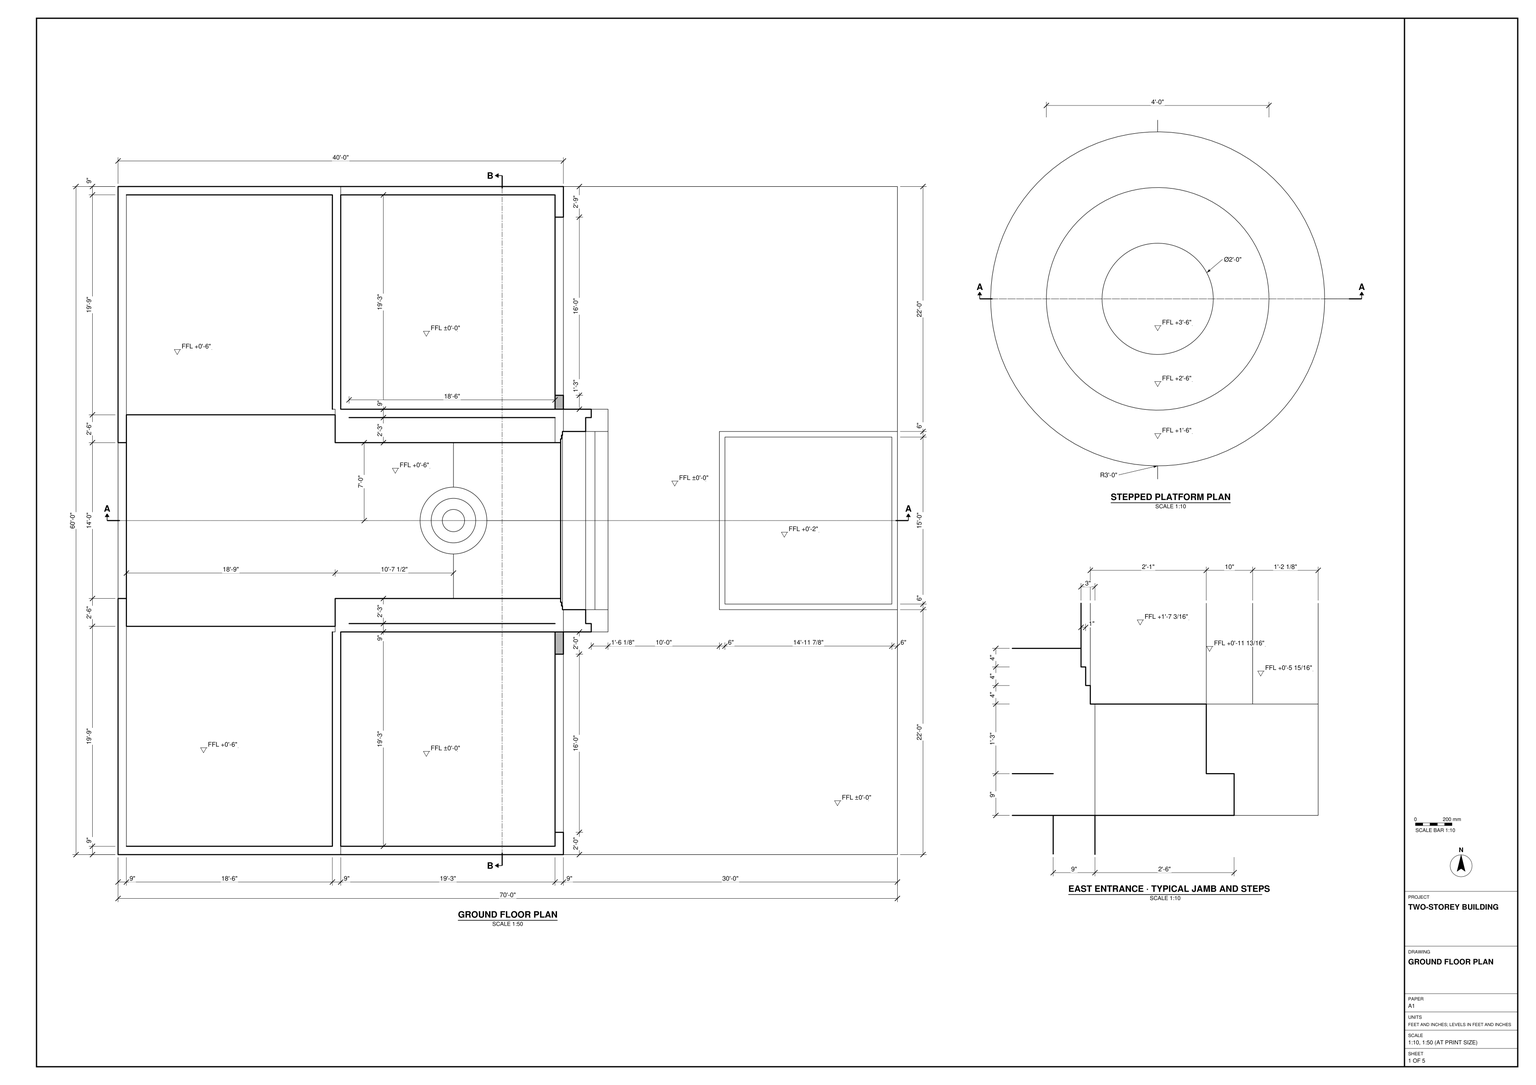
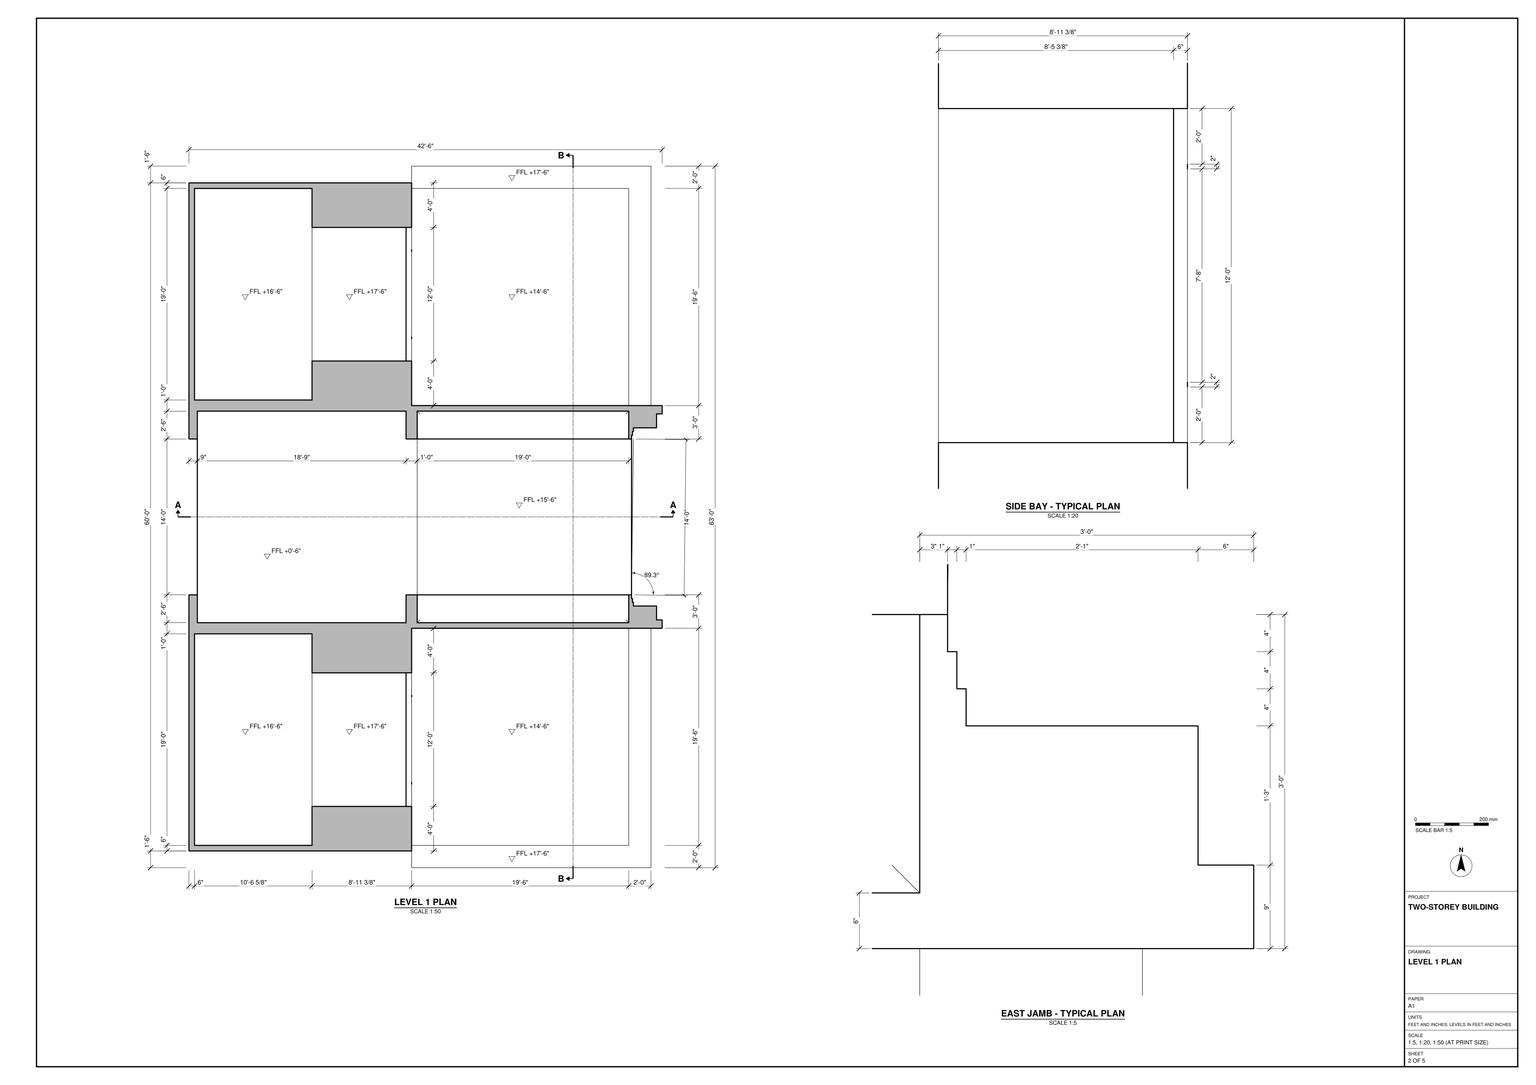
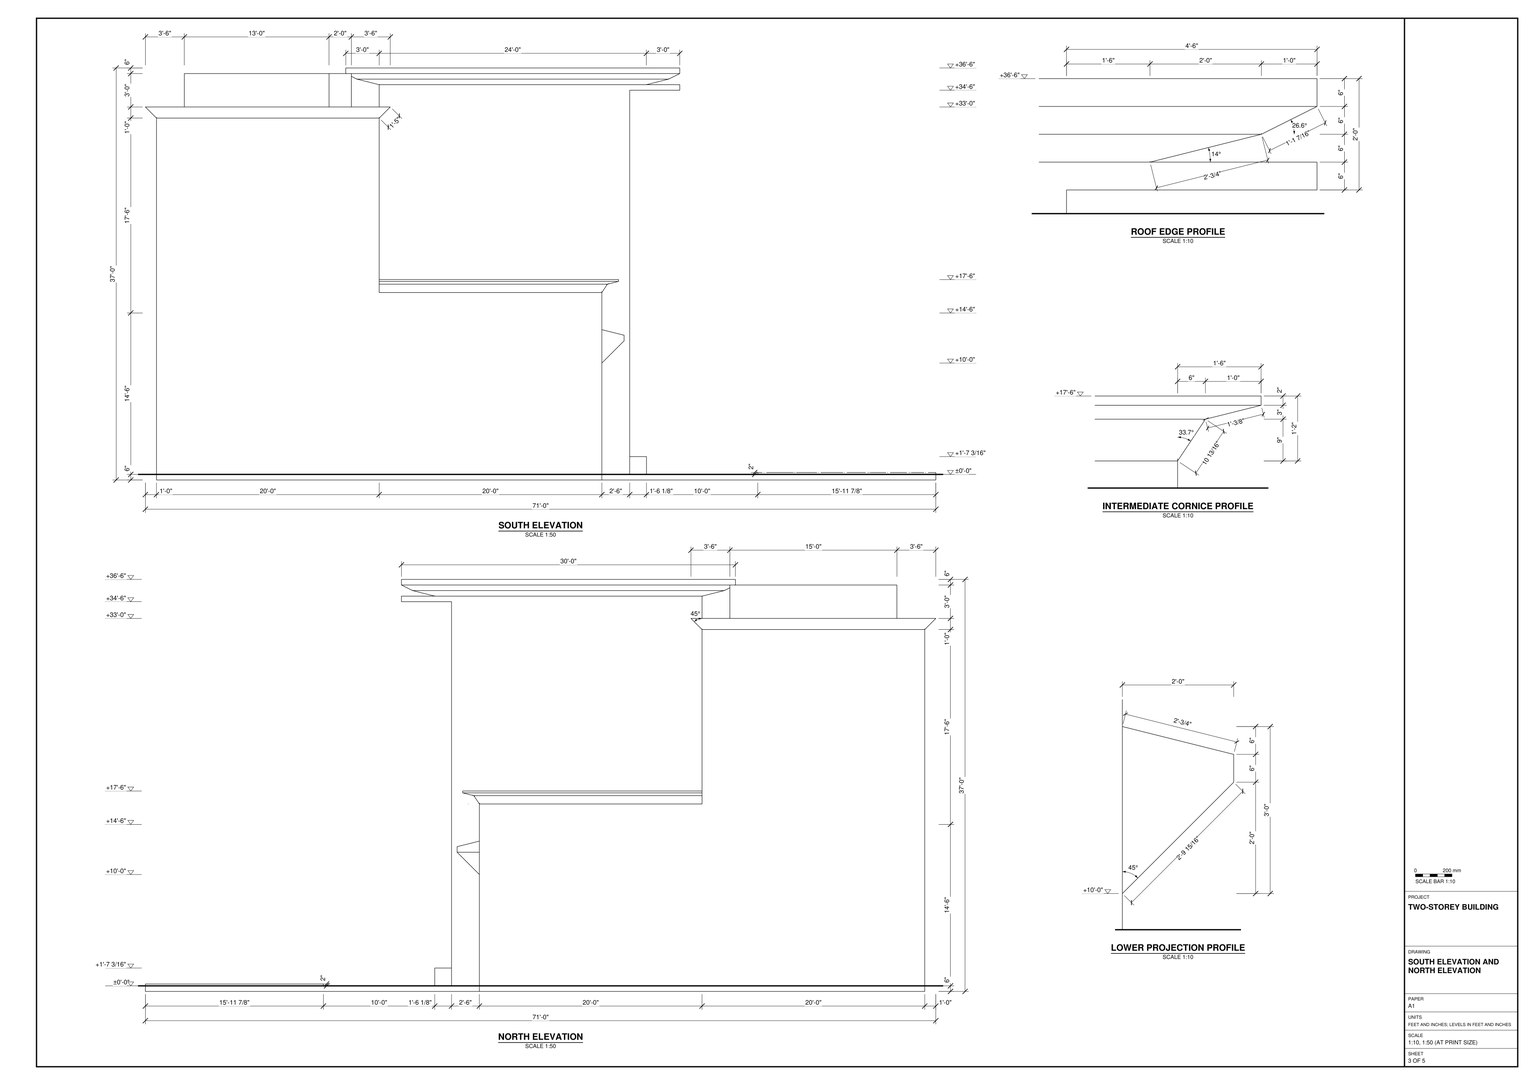
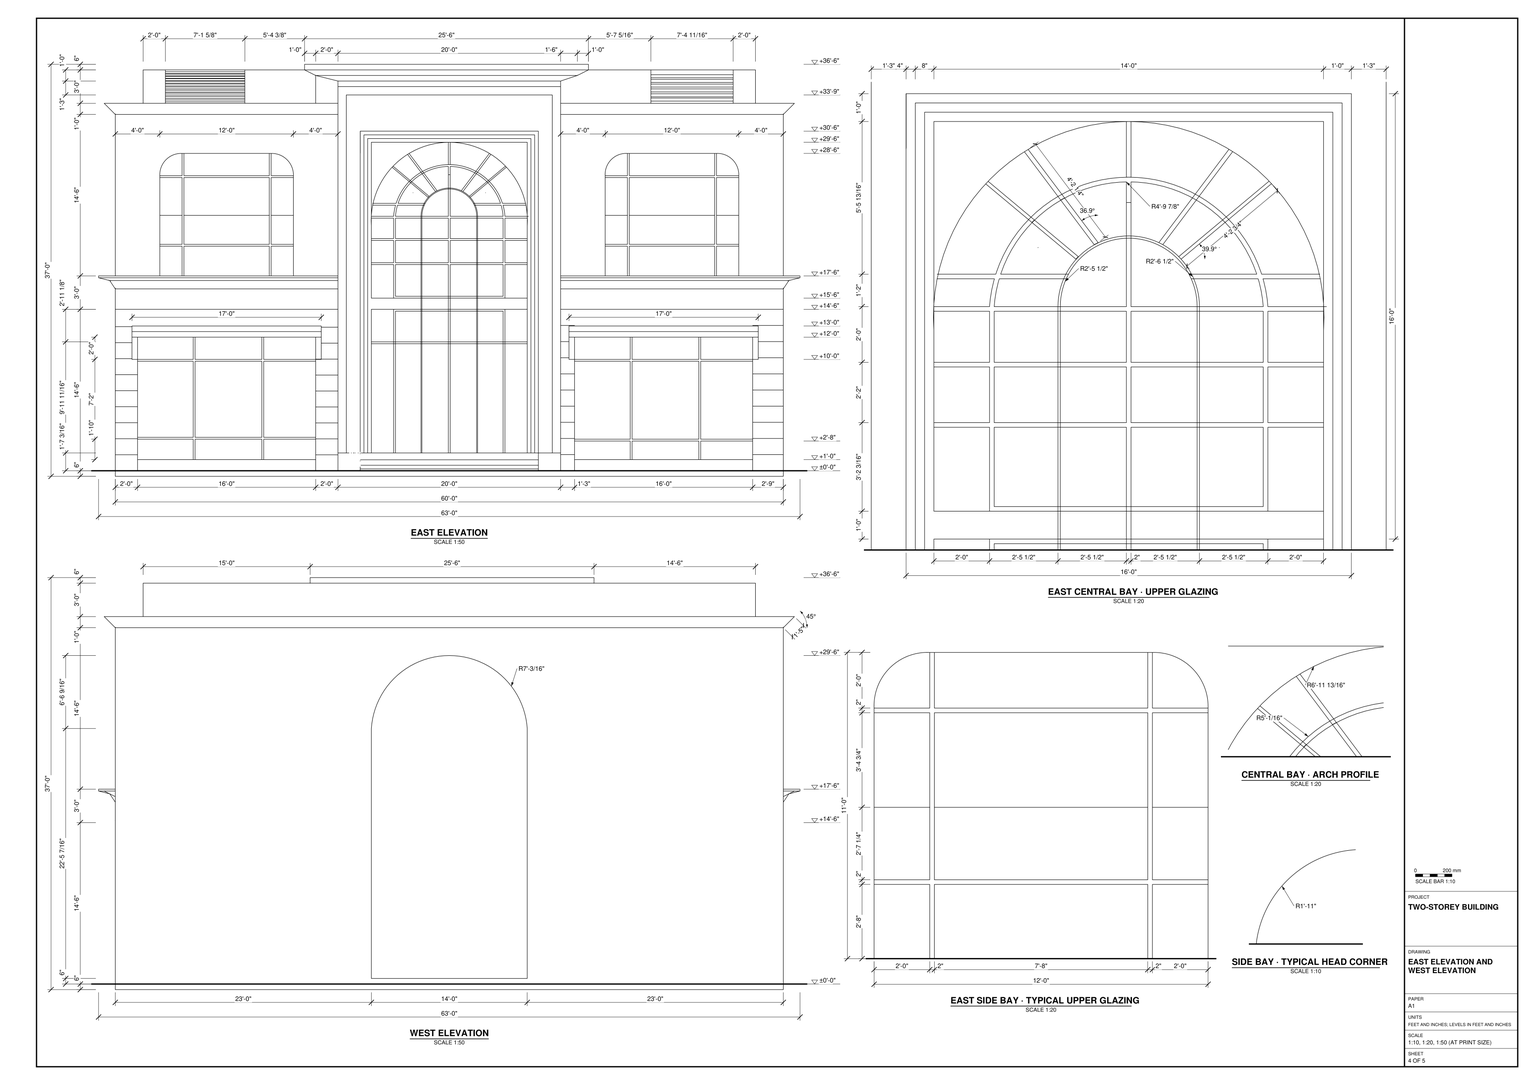
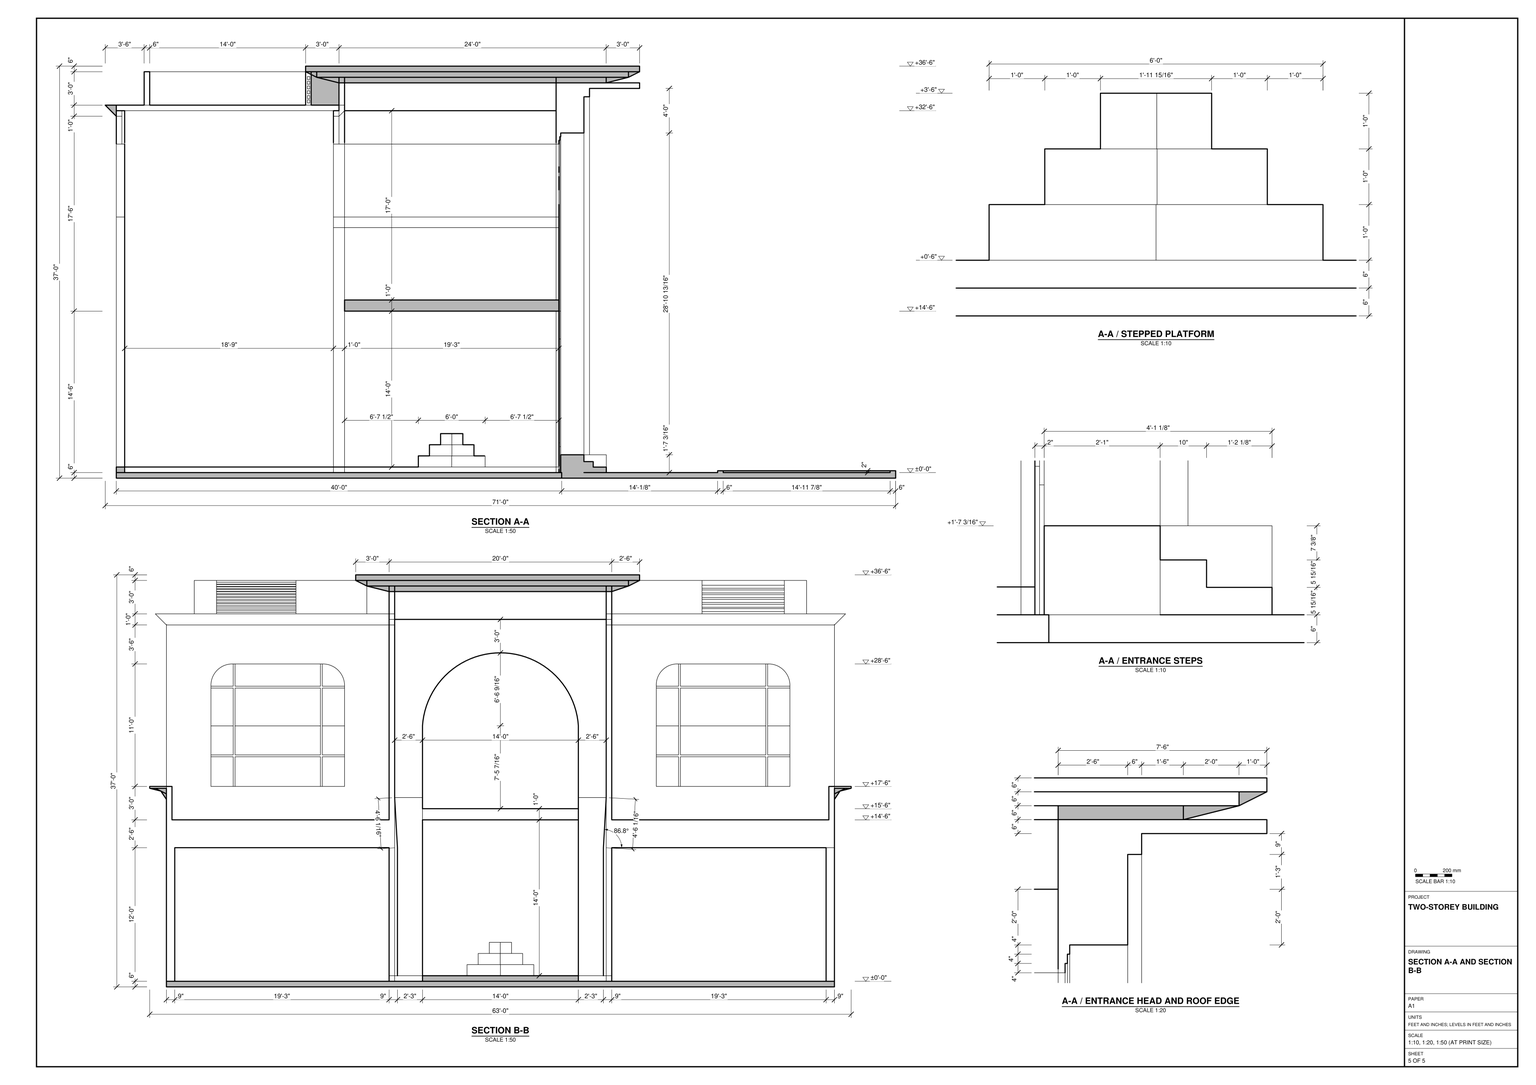
Build the two-storey building and its east forecourt in SketchUp using task_files/diagram_01.pdf. Work in feet and inches. The complete model shall measure 71'-0" east to west, 63'-0" north to south and 37'-0" from base to highest roof edge. Set the ground-floor datum at ±0'-0" and the upper-storey reference level at +14'-6". Follow the local floor levels marked on the plans rather than setting every slab on a storey at the same height.

Lay out the central east–west space with a pair of rooms on either side. Build the walls at their drawn thicknesses and retain the openings shown in plan. Align the concentric tiers of the circular platform with the east entrance. Model the entrance steps, profiled jambs and rectangular raised area across the forecourt. On the upper storey, distinguish the slab over the eastern part of the central space from the opening to the floor below. Follow the side-bay detail on both sides. Use the elevations and enlarged profiles to shape the roof edges, intermediate cornices and lower projections.

Keep walls, slabs, roof elements and each furniture or joinery piece shown in separate groups or components, and use components for repeated parts. Any decor or loose items shown may use suitable library components. Save one SketchUp model as output_files/two_storey_building_with_a_circular_stepped_platform.skp.

# SketchUp Ruby script. Lengths in inches.
U = 1.inch
M = Sketchup.active_model
def pt(a) = Geom::Point3d.new(a.map { |v| v * U })
def face(e, loops, mat)
  f = e.add_face(loops[0].map { |a| pt(a) })
  loops[1..].each { |l| e.add_face(l.map { |a| pt(a) }).erase! }
  f.material = f.back_material = mat if mat
  f
end
# faces: each face lists its corners as indices into pts; further lists are holes
def faces(e, pts, list, mat = nil) = list.each { |f| face(e, (f[0].is_a?(Array) ? f : [f]).map { |l| l.map { |i| pts[i] } }, mat) }
# xy, xz, yz: faces in a plane at the given z, y or x. An outline is a flat list of corners, or four numbers for a rectangle; further outlines are holes
def ring(l) = l.size == 4 ? [[l[0], l[1]], [l[2], l[1]], [l[2], l[3]], [l[0], l[3]]] : l.each_slice(2).to_a
def flat(e, list, mat, &to3) = list.each { |f| face(e, (f[0].is_a?(Array) ? f : [f]).map { |l| ring(l).map { |u, v| to3.(u, v) } }, mat) }
def xy(e, z, list, mat = nil) = flat(e, list, mat) { |x, y| [x, y, z] }
def xz(e, y, list, mat = nil) = flat(e, list, mat) { |x, z| [x, y, z] }
def yz(e, x, list, mat = nil) = flat(e, list, mat) { |y, z| [x, y, z] }
def lines(e, pts, list) = list.each { |a, b| e.add_line(pt(pts[a]), pt(pts[b])) }
# prism: a flat outline (further loops are holes) pulled along v
def prism(e, loops, v, mat = nil)
  f = face(e, loops, mat); d = Geom::Vector3d.new(v.map { |x| x * U })
  f.pushpull(f.normal.samedirection?(d) ? d.length : -d.length)
end
def box(e, o, s, mat = nil) = prism(e, [[o, [o[0] + s[0], o[1], o[2]], [o[0] + s[0], o[1] + s[1], o[2]], [o[0], o[1] + s[1], o[2]]]], [0, 0, s[2]], mat)
def at(x, y, z, deg = 0) = Geom::Transformation.translation(pt([x, y, z])) * Geom::Transformation.rotation(ORIGIN, Z_AXIS, deg.degrees)
def axes(o, x, y, z) = Geom::Transformation.new([*x, 0, *y, 0, *z, 0, *pt(o).to_a, 1])
def part(name) = M.definitions.add(name)
# library, detail: a bought-in or finely detailed component or shape, given as its bounding box
def library(name, o, s) = part(name).tap { |d| box(d.entities, o, s) }
def detail(e, o, s) = box(e.add_group.entities, o, s)
def put(e, d, t, mat = nil) = e.add_instance(d, t).tap { |i| i.material = mat if mat }
def group(e, t, mat = nil) = e.add_group.tap { |g| g.transformation = t; g.material = mat if mat }.entities
root = M.entities
M.materials.add("D01_Frost_White").color = [255, 242, 206]
M.materials.add("LightPink_Translucent").color = [144, 107, 117]
M.materials.add("ThomThom - Hat2").color = [38, 38, 38]
c1 = part("blade")
p = [[2.15,0.21,22],[0,0.17,0],[0.09,0.45,0],[2.18,0.31,22],[2.29,0.31,22],[0.38,0.45,0],
  [2.48,0.24,33],[2.49,0.24,33],[2.48,0.22,33]]
faces(c1.entities,p,[[0,1,2,3],[4,5,2,3],[6,3,4,7],[8,0,3,6]])
c2 = part("seeds")
p = [[0.3,-0.1,1.38],[-0.01,-0.03,1.59],[-0.01,-0.03,0.03],[0.14,-0.07,-0.07],[0.29,-0.03,3],[0.15,0.01,3.11]]
faces(c2.entities,p,[[0,1,2,3],[1,0,4,5]],"LightPink_Translucent")
c3 = part("blade with seeds")
put(c3.entities,c1,at(0,0,0))
put(c3.entities,c2,axes([2.4,0.25,30.99],[1.5799,-0.05474,1.17369],[-0.12525,1.92788,0.29478],[-0.07173,-0.02425,1.56792]))
c4 = part("Regal mist grass")
put(c4.entities,c3,axes([-3.26,-3.84,1.05],[0.05632,0.08194,0.78597],[-0.27153,0.73654,-0.07427],[-0.27499,0.00533,0.13909]))
put(c4.entities,c3,axes([-3.73,-1.59,0.19],[0.48504,-0.05875,0.50893],[-0.30767,0.51765,0.37393],[-0.23969,-0.07765,0.1121]))
put(c4.entities,c3,axes([-2.85,-2.28,0.11],[0.14833,0.22859,0.63362],[-0.3418,0.62134,-0.13627],[-0.35096,-0.14851,0.27091]))
put(c4.entities,c3,axes([3.2,1.81,0.97],[0.43228,0.51405,-0.15691],[-0.49359,0.48662,0.20258],[0.25079,0.07404,0.38762]))
put(c4.entities,c3,axes([2.7,2.1,0.19],[-0.42777,-0.23608,0.50893],[0.55235,-0.23987,0.37393],[0.14898,0.20319,0.1121]))
put(c4.entities,c3,axes([2.71,1.87,1.19],[0.04068,-0.83498,-0.05388],[0.77022,0.02282,-0.29906],[0.29664,0.058,0.45442]))
put(c4.entities,c3,axes([-3.45,-1.04,0.97],[-0.63139,-0.22904,-0.15691],[0.18416,-0.66822,0.20258],[-0.25421,0.06127,0.38762]))
put(c4.entities,c3,axes([-0.36,0.56,0.04],[0.20136,-0.97289,-0.10381],[0.95476,0.16959,0.22717],[-0.16683,-0.13435,0.69317]))
put(c4.entities,c3,axes([-2.43,-0.5,0.06],[0,0.82104,0.22],[-0.85,0,0],[0,-0.187,0.69788]))
put(c4.entities,c3,axes([1.82,-1.29,-0.13],[0.7903,0.13461,-0.27628],[-0.16677,0.83032,-0.07251],[0.23585,0.10061,0.60984]))
put(c4.entities,c3,axes([2.42,-3.36,0.01],[0.475,-0.82272,0],[0.79469,0.45881,-0.22867],[0.181,0.1045,0.72539]))
put(c4.entities,c3,axes([-2,3.05,0.45],[0.01669,-0.42385,0.68389],[0.75077,0.22388,0.09451],[-0.06505,0.45172,0.32293]))
put(c4.entities,c3,axes([-0.36,3.06,1.2],[-0.74862,-0.21464,0.23609],[0.25599,-0.70567,0.19467],[0.04499,0.27751,0.48853]))
put(c4.entities,c3,axes([-0.35,2.54,1.2],[0.22904,-0.63139,0.15691],[0.66822,0.18416,-0.20258],[0.06127,0.25421,0.38762]))
put(c4.entities,c3,axes([0.87,-4.07,1.06],[0.74862,0.21464,0.21269],[-0.25599,0.70567,0.17538],[-0.04499,-0.27751,0.44012]))
put(c4.entities,c3,axes([0.86,-3.55,1.2],[-0.22904,0.63139,0.15691],[-0.66822,-0.18416,-0.20258],[-0.06127,-0.25421,0.38762]))
put(c4.entities,c3,axes([-2.31,3.6875,0.11],[0.23975,-0.12952,0.63362],[0.59193,0.39053,-0.13627],[-0.17618,0.33792,0.27091]))
put(c4.entities,c3,axes([-0.89,-5.97,1.05],[-0.01417,0.09841,0.78597],[-0.69904,0.35716,-0.07427],[-0.20571,-0.18257,0.13909]))
put(c4.entities,c3,axes([2.82,2.98,-0.38],[0.05535,-0.11853,0.78135],[0.69686,-0.3491,-0.11937],[0.21127,0.18068,0.13309]))
put(c4.entities,c3,axes([0.6,3.36,1.05],[0.00225,-0.0994,0.78597],[0.65107,-0.43855,-0.07427],[0.22615,0.15653,0.13909]))
put(c4.entities,c3,axes([3.04,1.81,1.06],[-0.56019,0.541,0.21269],[-0.48313,-0.57453,0.17538],[0.26282,0.09979,0.44012]))
put(c4.entities,c3,axes([2.59,1.54,1.2],[-0.43228,-0.51405,0.15691],[0.49359,-0.48662,-0.20258],[0.25079,0.07404,0.38762]))
put(c4.entities,c3,axes([2.85,-2.86,-0.15],[0.71104,0.41052,-0.22],[-0.425,0.73612,0],[0.16194,0.0935,0.69788]))
put(c4.entities,c3,axes([-3.85,-0.6,1.05],[-0.12406,0.1066,0.77516],[0.01055,0.77884,-0.12259],[-0.28438,0.10128,0.06217]))
put(c4.entities,c3,axes([1.3,0.61,0.12],[0.56129,0.4933,0.06416],[-0.46819,0.55654,-0.18321],[-0.13032,0.07524,0.56159]))
put(c4.entities,c3,axes([1.125,0.43,0.14],[0.08853,0.93685,-0.12892],[-0.92207,0.05665,-0.22156],[-0.16237,0.12479,0.70765]))
put(c4.entities,c3,axes([-0.48,-0.93,-0.06],[0.36861,-0.73982,-0.19823],[0.76592,0.35605,0.0954],[0,-0.17054,0.63647]))
put(c4.entities,c3,axes([-3.05,-1.34,1.19],[0.38226,0.74345,-0.05388],[-0.67844,0.36535,-0.29906],[-0.2859,0.09809,0.45442]))
put(c4.entities,c3,axes([-0.85,-4.05,1.06],[0.3453,-0.52156,0.02849],[0.49172,0.30366,0.2243],[-0.15897,-0.16722,0.34202]))
put(c4.entities,c3,axes([-0.91,-3.46,1.17],[-0.64782,-0.39685,-0.31479],[0.4604,-0.69542,0.03799],[-0.23471,-0.23695,0.44531]))
put(c4.entities,c3,axes([5.64,-0.84,1.05],[0.10543,-0.12506,0.77516],[-0.13494,-0.76713,-0.12259],[0.26452,-0.14545,0.06217]))
put(c4.entities,c3,axes([0.86,-0.73,-0.0625],[0,-0.95,0],[0.95,0,0],[0,0,0.79515]))
put(c4.entities,c3,axes([1.65,0.49,0.68],[-0.2822,-0.14146,0.75935],[0.58401,-0.59344,0.0614],[0.36399,0.26771,0.32462]))
put(c4.entities,c3,axes([3.38,1.37,1.05],[0.16298,-0.01389,0.77516],[0.44703,-0.63786,-0.12259],[0.28989,0.0842,0.06217]))
put(c4.entities,c3,axes([3.82,0.11,1.06],[-0.21464,0.74862,0.21269],[-0.70567,-0.25599,0.17538],[0.27751,-0.04499,0.44012]))
put(c4.entities,c3,axes([3.3,0.1,1.2],[-0.63139,-0.22904,0.15691],[0.18416,-0.66822,-0.20258],[0.25421,-0.06127,0.38762]))
put(c4.entities,c3,axes([0.07,2.77,1.03],[0.74683,0.20582,-0.22641],[-0.25599,0.70567,-0.17538],[0.06848,0.28411,0.43322]))
put(c4.entities,c3,axes([-0.56,3.11,1.06],[-0.55982,0.27904,0.02849],[-0.27401,-0.50883,0.2243],[0.05406,0.2243,0.34202]))
put(c4.entities,c3,axes([-0.21,2.64,1.17],[0.36261,0.66759,-0.31479],[-0.74642,0.37205,0.03799],[0.08479,0.32256,0.44531]))
put(c4.entities,c3,axes([0.99,-1.65,0.12],[0.14656,-0.73274,0.06416],[0.71607,0.12719,-0.18321],[0.13032,0.07524,0.56159]))
put(c4.entities,c3,axes([1.74,-2.51,0.06],[-0.81639,0.21792,0.07817],[-0.20159,-0.81098,0.15546],[0.07281,0.11816,0.71074]))
put(c4.entities,c3,axes([1.48,-0.78,0.16],[0.36861,-0.73982,0.19823],[0.76592,0.35605,-0.0954],[0,0.17054,0.63647]))
put(c4.entities,c3,axes([0.64,1.03,0.43],[0.65653,0.33108,0.67022],[-0.64318,0.71325,0.26504],[-0.28809,-0.42273,0.56186]))
put(c4.entities,c3,axes([-3.14,0.74,1.06],[-0.18842,-0.75564,0.21269],[0.73912,-0.13114,0.17538],[-0.21784,0.17772,0.44012]))
put(c4.entities,c3,axes([-3.22,0.89,0.97],[-0.66132,0.11734,-0.15691],[-0.17463,-0.67077,0.20258],[-0.18951,0.18017,0.38762]))
put(c4.entities,c3,axes([-2.23,-2.48,1.17],[-0.75946,-0.01977,-0.31479],[0.05101,-0.83245,0.03799],[-0.32174,-0.08785,0.44531]))
put(c4.entities,c3,axes([-2.76,-3.02,1.22],[0.62742,-0.60592,0.23822],[0.54111,0.64347,0.19642],[-0.29436,-0.11177,0.49293]))
put(c4.entities,c3,axes([-2.08,-2.56,1.2],[0.43228,0.51405,0.15691],[-0.49359,0.48662,-0.20258],[-0.25079,-0.07404,0.38762]))
put(c4.entities,c3,axes([1.55,-0.55,0.14],[0.8556,0.39175,-0.12892],[-0.41198,0.82685,-0.22156],[0.02689,0.20301,0.70765]))
put(c4.entities,c3,axes([1.48,-0.16,-0.06],[0.53033,0.53033,0],[-0.53033,0.53033,0],[0,0,0.75]))
put(c4.entities,c3,axes([2.63,-2.96,1.19],[-0.83498,-0.04068,-0.05388],[0.02282,-0.77022,-0.29906],[0.058,-0.29664,0.45442]))
put(c4.entities,c3,axes([2.0625,-3.25,1.03],[-0.54387,-0.55166,-0.22641],[0.57453,-0.48313,-0.17538],[0.08275,-0.28029,0.43322]))
put(c4.entities,c3,axes([3.97,0.02,0.97],[0.63139,0.22904,-0.15691],[-0.18416,0.66822,0.20258],[0.25421,-0.06127,0.38762]))
put(c4.entities,c3,axes([4.49,1.89,0.7],[-0.14541,-0.69018,-0.01547],[0.68728,-0.15867,-0.07015],[0.14352,0.04375,0.23137]))
put(c4.entities,c3,axes([3.57,0.32,1.19],[-0.38226,-0.74345,-0.05388],[0.67844,-0.36535,-0.29906],[0.2859,-0.09809,0.45442]))
put(c4.entities,c3,axes([-1.14,-3.99,0.97],[-0.11734,-0.66132,-0.15691],[0.67077,-0.17463,0.20258],[-0.18017,-0.18951,0.38762]))
put(c4.entities,c3,axes([-0.04,-4.56,-0.1],[-0.52501,0.47102,-0.01725],[-0.48105,-0.51587,-0.0782],[-0.03387,-0.14617,0.25794]))
put(c4.entities,c3,axes([-0.69,-4.1,1.37],[-0.50704,0.78711,-0.06035],[-0.7343,-0.45346,-0.33495],[-0.25525,-0.22238,0.50895]))
put(c4.entities,c3,axes([-1.22,-3.44,1.03],[-0.74969,0.19517,-0.22641],[-0.13114,-0.73912,-0.17538],[-0.20136,-0.21181,0.43322]))
put(c4.entities,c3,axes([3.39,-4.18,1.05],[-0.00733,-0.1634,0.77516],[-0.61941,-0.47227,-0.12259],[0.09577,-0.28628,0.06217]))
put(c4.entities,c3,axes([-2.27,-0.88,-0.01],[-0.70668,0.69027,0.13628],[-0.70711,-0.68301,-0.16169],[-0.02468,-0.19603,0.73059]))
put(c4.entities,c3,axes([-0.42,0.16,-0.06],[-0.4564,-0.68913,-0.19823],[0.69131,-0.48528,0.0954],[-0.14769,-0.08527,0.63647]))
put(c4.entities,c3,axes([-1.79,1.83,1.2],[0.51405,-0.43228,0.15691],[0.48662,0.49359,-0.20258],[-0.07404,0.25079,0.38762]))
put(c4.entities,c3,axes([-2.14,3.0625,0.21],[0.69018,-0.14539,0.02883],[0.15867,0.58575,-0.38241],[-0.04375,0.29652,0.34277]))
put(c4.entities,c3,axes([-0.57,2.8,1.19],[0.74345,-0.38226,-0.05388],[0.36535,0.67844,-0.29906],[0.09809,0.2859,0.45442]))
put(c4.entities,c3,axes([-2.68,0.49,1.2],[0.66132,-0.11734,0.15691],[0.17463,0.67077,-0.20258],[-0.18951,0.18017,0.38762]))
put(c4.entities,c3,axes([-2.06,2.27,1.06],[-0.541,-0.56019,0.21269],[0.57453,-0.48313,0.17538],[-0.09979,0.26282,0.44012]))
put(c4.entities,c3,axes([1.29,-3.38,0.68],[-0.14146,0.2822,0.75935],[-0.59344,-0.58401,0.0614],[0.26771,-0.36399,0.32462]))
put(c4.entities,c3,axes([3.8,-1.61,1.06],[0.52156,0.3453,0.02849],[-0.30366,0.49172,0.2243],[0.16722,-0.15897,0.34202]))
put(c4.entities,c3,axes([3.21,-1.68,1.17],[0.39685,-0.64782,-0.31479],[0.69542,0.4604,0.03799],[0.23695,-0.23471,0.44531]))
put(c4.entities,c3,axes([4.29,-0.11,-0.16],[-0.48932,0.09853,0.62734],[-0.07789,-0.78429,0.03591],[0.34272,-0.11871,0.35698]))
put(c4.entities,c3,axes([-0.57,-0.3125,0.14],[-0.8556,-0.39175,-0.12892],[0.41198,-0.82685,-0.22156],[-0.02689,-0.20301,0.70765]))
put(c4.entities,c3,axes([-3.375,-0.75,-0.38],[0.01927,0.12939,0.78135],[-0.38842,0.67573,-0.11937],[-0.2759,-0.03406,0.13309]))
put(c4.entities,c3,axes([-3.83,2.3125,1.05],[-0.01889,0.16248,0.77516],[0.53593,0.56522,-0.12259],[-0.1403,0.26729,0.06217]))
put(c4.entities,c3,axes([-5.23,0.19,1.05],[0.09696,0.02202,0.78597],[0.29994,0.72543,-0.07427],[-0.19848,0.1904,0.13909]))
put(c4.entities,c3,axes([-1.08,-3.5625,0.01],[-0.475,-0.82272,0],[0.79469,-0.45881,-0.22867],[0.181,-0.1045,0.72539]))
put(c4.entities,c3,axes([-0.27,-3.37,-0.14],[0.70879,0.20315,-0.13726],[-0.17846,0.71541,0.13726],[0.14289,-0.0825,0.61578]))
put(c4.entities,c3,axes([3.53,-0.32,1.03],[0.20582,-0.74683,-0.22641],[0.70567,0.25599,-0.17538],[0.28411,-0.06848,0.43322]))
put(c4.entities,c3,axes([2.25,-0.8,0.68],[-0.31513,0.0186,0.75935],[0.20905,-0.80594,0.0614],[0.44908,0.04985,0.32462]))
put(c4.entities,c3,axes([3.875,0.31,1.06],[0.27904,0.55982,0.02849],[-0.50883,0.27401,0.2243],[0.2243,-0.05406,0.34202]))
put(c4.entities,c3,axes([3.4,-0.04,1.17],[0.66759,-0.36261,-0.31479],[0.37205,0.74642,0.03799],[0.32256,-0.08479,0.44531]))
put(c4.entities,c3,axes([-2.2,-2.88,1.19],[-0.04068,0.83498,-0.05388],[-0.77022,-0.02282,-0.29906],[-0.29664,-0.058,0.45442]))
put(c4.entities,c3,axes([-2.49,-2.3125,1.03],[-0.55166,0.54387,-0.22641],[-0.48313,-0.57453,-0.17538],[-0.28029,-0.08275,0.43322]))
put(c4.entities,c3,axes([0.49,1.3125,0.68],[-0.17367,-0.26361,0.75935],[0.80249,-0.22193,0.0614],[0.18137,0.41384,0.32462]))
put(c4.entities,c3,axes([-2.47,-3.02,1.06],[0.03826,-0.62433,0.02849],[0.57767,0.01712,0.2243],[-0.22128,-0.06533,0.34202]))
put(c4.entities,c3,axes([0.09,-5.13,-0.38],[-0.12743,0.02958,0.78135],[-0.70471,-0.33298,-0.11937],[0.01182,-0.27774,0.13309]))
put(c4.entities,c3,axes([1.8,-0.61,0.12],[0.70785,-0.23944,0.06416],[0.24789,0.68373,-0.18321],[0,0.15048,0.56159]))
put(c4.entities,c3,axes([2.92,-0.39,0.06],[-0.59691,-0.59805,0.07817],[0.60154,-0.58007,0.15546],[-0.06593,0.12214,0.71074]))
put(c4.entities,c3,axes([2.77,-3.23,1.06],[0.62433,0.03826,0.02849],[-0.01712,0.57767,0.2243],[0.06533,-0.22128,0.34202]))
put(c4.entities,c3,axes([-0.93,1.44,0.68],[-0.0186,-0.31513,0.75935],[0.80594,0.20905,0.0614],[-0.04985,0.44908,0.32462]))
put(c4.entities,c3,axes([2.23,-3,1.17],[0.01977,-0.75946,-0.31479],[0.83245,0.05101,0.03799],[0.08785,-0.32174,0.44531]))
put(c4.entities,c3,axes([-2.22,0.85,0.68],[0.14146,-0.2822,0.75935],[0.59344,0.58401,0.0614],[-0.26771,0.36399,0.32462]))
put(c4.entities,c3,axes([2.57,-3.29,1.06],[0.541,0.56019,0.21269],[-0.57453,0.48313,0.17538],[0.09979,-0.26282,0.44012]))
put(c4.entities,c3,axes([-0.83,0.43,-0.13],[-0.7903,-0.13461,-0.27628],[0.16677,-0.83032,-0.07251],[-0.23585,-0.10061,0.60984]))
put(c4.entities,c3,axes([1.17,1.85,0.11],[0.01341,-0.27217,0.63362],[0.64069,-0.30401,-0.13627],[0.19778,0.32575,0.27091]))
put(c4.entities,c3,axes([-3.05,-0.3125,0.68],[0.26361,-0.17367,0.75935],[0.22193,0.80249,0.0614],[-0.41384,0.18137,0.32462]))
put(c4.entities,c3,axes([0.55,4.79,1.46],[0.52501,-0.47102,-0.02875],[0.48105,0.51587,-0.13034],[0.03387,0.14617,0.4299]))
put(c4.entities,c3,axes([1.19,2.78,1.19],[0.45272,-0.70277,-0.05388],[0.65562,0.40488,-0.29906],[0.2279,0.19855,0.45442]))
put(c4.entities,c3,axes([3.41,0.38,-0.14],[-0.53033,0.51226,-0.13726],[-0.53033,-0.51226,0.13726],[0,0.165,0.61578]))
put(c4.entities,c3,axes([1.4,-1.03,-0.06],[0.4564,0.68913,-0.19823],[-0.69131,0.48528,0.0954],[0.14769,0.08527,0.63647]))
put(c4.entities,c3,axes([-4.42,2.5,0.19],[0.31662,-0.37211,0.50893],[0.12494,0.58908,0.37393],[-0.22881,0.10548,0.1121]))
put(c4.entities,c3,axes([2.01,-2.93,0.06],[-0.71104,-0.41052,0.22],[0.425,-0.73612,0],[0.16194,0.0935,0.69788]))
put(c4.entities,c3,axes([-2.08,0.23,0.68],[0.18976,-0.25227,0.75935],[0.47913,0.68094,0.0614],[-0.32863,0.3101,0.32462]))
put(c4.entities,c3,axes([-3.03,0.43,1.19],[0.70277,0.45272,-0.05388],[-0.40488,0.65562,-0.29906],[-0.19855,0.2279,0.45442]))
put(c4.entities,c3,axes([1.41,2.83,-0.15],[-0.71104,0.41052,-0.22],[-0.425,-0.73612,0],[-0.16194,0.0935,0.69788]))
put(c4.entities,c3,axes([0.92,0.8,0.05],[-0.74186,-0.66083,-0.11162],[0.62425,-0.74205,0.24427],[-0.19977,0.0773,0.74534]))
put(c4.entities,c3,axes([1.1,0,-0.02],[-0.70668,-0.70668,-0.02717],[0.70711,-0.70711,0],[-0.02468,-0.02468,0.77794]))
put(c4.entities,c3,axes([-2.8,-1.26,-0.15],[0,-0.82104,-0.22],[0.85,0,0],[0,-0.187,0.69788]))
put(c4.entities,c3,axes([1.34,-0.35,-0.02],[0,0.94953,-0.02498],[-0.95,0,0],[0,0.02984,0.79476]))
put(c4.entities,c3,axes([2.98,2.01,1.06],[-0.03826,0.62433,0.02849],[-0.57767,-0.01712,0.2243],[0.22128,0.06533,0.34202]))
put(c4.entities,c3,axes([-1.42,-3.85,0.68],[0.17367,0.26361,0.75935],[-0.80249,0.22193,0.0614],[-0.18137,-0.41384,0.32462]))
put(c4.entities,c3,axes([2.75,1.47,1.17],[0.75946,0.01977,-0.31479],[-0.05101,0.83245,0.03799],[0.32174,0.08785,0.44531]))
put(c4.entities,c3,axes([-0.4375,2.95,-0.38],[0.12296,-0.04468,0.78135],[0.7396,0.2459,-0.11937],[0.02163,0.27715,0.13309]))
put(c4.entities,c3,axes([1.25,2.43,1.2],[-0.11734,-0.66132,0.15691],[0.67077,-0.17463,-0.20258],[0.18017,0.18951,0.38762]))
put(c4.entities,c3,axes([1.46,2.61,-0.07],[-0.46908,-0.8256,-0.02278],[0.79469,-0.45881,0.22867],[-0.19583,0.0786,0.72503]))
put(c4.entities,c3,axes([1.48,2.1875,-0.01],[0.95113,0.26686,0.13628],[-0.23795,0.95388,-0.16169],[-0.15742,0.11938,0.73059]))
put(c4.entities,c3,axes([1.71,-1.37,0.94],[-0.65649,-0.4266,0.61271],[0.6932,-0.66419,0.26437],[0.21181,0.40027,0.59225]))
put(c4.entities,c3,axes([3.61,0.25,-0.07],[-0.94953,-0.00656,-0.02205],[0,-0.91763,0.22129],[-0.02984,0.20889,0.70164]))
put(c4.entities,c3,axes([-1.67,1.69,-0.14],[-0.17846,-0.71541,-0.13726],[0.70879,-0.20315,0.13726],[-0.14289,-0.0825,0.61578]))
put(c4.entities,c3,axes([-2.12,1.95,1.35],[0.83498,0.04068,-0.05981],[-0.02282,0.77022,-0.33196],[-0.058,0.29664,0.5044]))
put(c4.entities,c3,axes([-3.28,0.6,1.06],[-0.52156,-0.3453,0.02849],[0.30366,-0.49172,0.2243],[-0.16722,0.15897,0.34202]))
put(c4.entities,c3,axes([-2.68,0.97,1.03],[0.19517,0.74969,-0.22641],[-0.73912,0.13114,-0.17538],[-0.21181,0.20136,0.43322]))
put(c4.entities,c3,axes([-3.02,-0.7,1.03],[-0.20582,0.74683,-0.22641],[-0.70567,-0.25599,-0.17538],[-0.28411,0.06848,0.43322]))
put(c4.entities,c3,axes([-0.75,4.32,1.05],[0.0963,0.13221,0.77516],[0.77718,0.05194,-0.12259],[0.07815,0.29158,0.06217]))
put(c4.entities,c3,axes([-0.25,0.09,0.01],[0.96024,0.17298,0.20273],[-0.19542,0.97698,0.07956],[-0.14033,-0.09434,0.70387]))
put(c4.entities,c3,axes([3.41,-0.36,0.06],[0,-0.82104,0.22],[0.85,0,0],[0,0.187,0.69788]))
put(c4.entities,c3,axes([1.46,0.0625,-0.06],[-0.36861,0.73982,-0.19823],[-0.76592,-0.35605,0.0954],[0,0.17054,0.63647]))
put(c4.entities,c3,axes([-2.58,-3.03,0.68],[0.2822,0.14146,0.75935],[-0.58401,0.59344,0.0614],[-0.36399,-0.26771,0.32462]))
put(c4.entities,c3,axes([5.27,-1.64,1.05],[-0.09923,-0.00624,0.78597],[-0.41207,-0.66814,-0.07427],[0.16548,-0.21969,0.13909]))
put(c4.entities,c3,axes([-1.55,2.24,1.18],[0.54387,0.55166,-0.25132],[-0.57453,0.48313,-0.19467],[-0.08275,0.28029,0.48087]))
put(c4.entities,c3,axes([-2.06,2.44,0.97],[-0.51405,0.43228,-0.15691],[-0.48662,-0.49359,0.20258],[-0.07404,0.25079,0.38762]))
put(c4.entities,c3,axes([-1.87,2,-0.15],[-0.71104,-0.41052,-0.22],[0.425,-0.73612,0],[-0.16194,-0.0935,0.69788]))
put(c4.entities,c3,axes([5.09,2.53,1.05],[-0.0687,-0.07188,0.78597],[0.15027,-0.77048,-0.07427],[0.2706,-0.04923,0.13909]))
put(c4.entities,c3,axes([0.88,1.48,-0.02],[0.33031,0.94323,-0.02664],[-0.9438,0.33051,0],[0.01153,0.03294,0.76288]))
put(c4.entities,c3,axes([1.39,1.36,-0.07],[0.79762,-0.27858,-0.08506],[0.28027,0.80246,0.00004],[0.08804,-0.03079,0.77052]))
put(c4.entities,c3,axes([5.31,0.16,0.19],[-0.46941,0.13554,0.50893],[0.22095,-0.56018,0.37393],[0.24902,0.03833,0.1121]))
put(c4.entities,c3,axes([0.46,1.46,-0.0625],[-0.24789,-0.70785,0],[0.70785,-0.24789,0],[0,0,0.684]))
put(c4.entities,c3,axes([1.71,-4.23,0.11],[-0.21596,0.16619,0.63362],[-0.64676,-0.29087,-0.13627],[0.11989,-0.36174,0.27091]))
put(c4.entities,c3,axes([1.16,1.79,-0.0625],[0.76592,0.36861,0],[-0.36861,0.76592,0],[0,0,0.7752]))
put(c4.entities,c3,axes([3.79,-2.27,0.11],[-0.27141,-0.02432,0.63362],[-0.27805,-0.65237,-0.13627],[0.33343,-0.18455,0.27091]))
put(c4.entities,c3,axes([4.82,-0.62,-0.38],[-0.03971,-0.12465,0.78135],[0.27539,-0.72914,-0.11937],[0.27779,-0.01049,0.13309]))
put(c4.entities,c3,axes([1.09,-3.82,1.19],[-0.74345,0.38226,-0.05388],[-0.36535,-0.67844,-0.29906],[-0.09809,-0.2859,0.45442]))
put(c4.entities,c3,axes([0.45,-3.79,1.03],[-0.74683,-0.20582,-0.22641],[0.25599,-0.70567,-0.17538],[-0.06848,-0.28411,0.43322]))
put(c4.entities,c3,axes([1.07,-4.125,1.06],[0.55982,-0.27904,0.02849],[0.27401,0.50883,0.2243],[-0.05406,-0.2243,0.34202]))
put(c4.entities,c3,axes([0.72,-3.65,1.17],[-0.36261,-0.66759,-0.31479],[0.74642,-0.37205,0.03799],[-0.08479,-0.32256,0.44531]))
put(c4.entities,c3,axes([0.55,0.66,-0.06],[-0.82501,0.05068,-0.19823],[-0.07461,-0.84133,0.0954],[-0.14769,0.08527,0.63647]))
put(c4.entities,c3,axes([-1.4375,2.49,0.01],[-0.475,0.82272,0],[-0.79469,-0.45881,-0.22867],[-0.181,-0.1045,0.72539]))
put(c4.entities,c3,axes([2.06,2.7,0.01],[0.475,0.82272,0],[-0.79469,0.45881,-0.22867],[-0.181,0.1045,0.72539]))
put(c4.entities,c3,axes([1.25,2.5,-0.14],[-0.70879,-0.20315,-0.13726],[0.17846,-0.71541,0.13726],[-0.14289,0.0825,0.61578]))
put(c4.entities,c3,axes([-4.18,2.4,1.46],[0.67042,0.21916,-0.02875],[-0.20623,0.67454,-0.13034],[-0.10965,0.10242,0.4299]))
put(c4.entities,c3,axes([-1.87,-4.98,0.19],[0.39631,0.28576,0.50893],[-0.57716,0.17178,0.37393],[-0.12349,-0.21962,0.1121]))
put(c4.entities,c3,axes([-1.64,-4.54,0.11],[-0.04601,0.26859,0.63362],[-0.67257,0.22484,-0.13627],[-0.15721,-0.34715,0.27091]))
put(c4.entities,c3,axes([-3.36,-1.32,1.06],[-0.27904,-0.55982,0.02849],[0.50883,-0.27401,0.2243],[-0.2243,0.05406,0.34202]))
put(c4.entities,c3,axes([-0.3,-1.11,0.16],[-0.82501,0.05068,0.19823],[-0.07461,-0.84133,-0.0954],[0.14769,-0.08527,0.63647]))
put(c4.entities,c3,axes([0.41,-1.33,0.01],[-0.62993,0.7451,0.20273],[-0.74838,-0.65773,0.07956],[0.15186,-0.07436,0.70387]))
put(c4.entities,c3,axes([0.41,-2.01,-0.13],[0.51173,-0.61712,-0.27628],[0.63569,0.55959,-0.07251],[0.20505,-0.15394,0.60984]))
put(c4.entities,c3,axes([-1.53,-1.15,0.44],[0.21595,-0.11877,0.78455],[0.07447,0.82927,0.0614],[-0.46776,0.11004,0.2804]))
put(c4.entities,c3,axes([1.65,-0.55,0.22],[-0.02075,-0.77304,0.62596],[0.93928,0.20038,0.26504],[-0.22215,0.423,0.59086]))
put(c4.entities,c3,axes([-0.15,-1.29,0.14],[-0.08853,-0.93685,-0.12892],[0.92207,-0.05665,-0.22156],[0.16237,-0.12479,0.70765]))
put(c4.entities,c3,axes([-0.43,-3.69,-0.15],[0.71104,-0.41052,-0.22],[0.425,0.73612,0],[0.16194,-0.0935,0.69788]))
put(c4.entities,c3,axes([5.18,-0.8,-0.04],[-0.47102,-0.52501,-0.02875],[0.51587,-0.48105,-0.13034],[0.14617,-0.03387,0.4299]))
put(c4.entities,c3,axes([3.54,-1.44,1.19],[-0.70277,-0.45272,-0.05388],[0.40488,-0.65562,-0.29906],[0.19855,-0.2279,0.45442]))
put(c4.entities,c3,axes([3.19,-1.98,1.03],[-0.19517,-0.74969,-0.22641],[0.73912,-0.13114,-0.17538],[0.21181,-0.20136,0.43322]))
put(c4.entities,c3,axes([4.43,1.06,0.11],[-0.18297,-0.20193,0.63362],[0.23807,-0.668,-0.13627],[0.37019,0.09049,0.27091]))
put(c4.entities,c3,axes([3.74,-1.9,0.97],[0.66132,-0.11734,-0.15691],[0.17463,0.67077,0.20258],[0.18951,-0.18017,0.38762]))
put(c4.entities,c3,axes([-3.89,3.98,1.05],[0.08619,-0.04957,0.78597],[0.71239,0.32972,-0.07427],[-0.01674,0.27453,0.13909]))
put(c4.entities,c3,axes([-1.73,4.12,0.19],[-0.01966,-0.48819,0.50893],[0.49131,0.3482,0.37393],[-0.09662,0.23269,0.1121]))
put(c4.entities,c3,axes([-3.18,-1.73,0.68],[0.31513,-0.0186,0.75935],[-0.20905,0.80594,0.0614],[-0.44908,-0.04985,0.32462]))
put(c4.entities,c3,axes([1.73,2.43,1.03],[0.74969,-0.19517,-0.22641],[0.13114,0.73912,-0.17538],[0.20136,0.21181,0.43322]))
put(c4.entities,c3,axes([1.36,3.03,1.06],[-0.3453,0.52156,0.02849],[-0.49172,-0.30366,0.2243],[0.15897,0.16722,0.34202]))
put(c4.entities,c3,axes([2.76,3.18,0.14],[-0.48719,-0.02575,0.46551],[0.32174,-0.54689,0.25702],[0.19246,0.1943,0.36515]))
put(c4.entities,c3,axes([-0.01,0.79,0.12],[-0.14656,0.73274,0.06416],[-0.71607,-0.12719,-0.18321],[-0.13032,-0.07524,0.56159]))
put(c4.entities,c3,axes([0.68,-1.46,0.16],[-0.4564,-0.68913,0.19823],[0.69131,-0.48528,-0.0954],[0.14769,0.08527,0.63647]))
put(c4.entities,c3,axes([1.23,-0.95,0.02],[-0.96024,-0.17298,0.21799],[0.19542,-0.97698,0.08554],[0.14033,0.09434,0.75685]))
put(c4.entities,c3,axes([-0.5,-0.09,0.16],[-0.36861,0.73982,0.19823],[-0.76592,-0.35605,-0.0954],[0,-0.17054,0.63647]))
put(c4.entities,c3,axes([4.1,-3.47,0.19],[-0.25305,0.41795,0.50893],[-0.21751,-0.56153,0.37393],[0.209,-0.14071,0.1121]))
put(c4.entities,c3,axes([1.9,0.29,-0.11],[0.27858,0.75173,-0.30667],[-0.80246,0.27073,-0.08049],[0.03079,0.25455,0.67692]))
put(c4.entities,c3,axes([3.99,-0.22,0.01],[0.95,0,0],[0,0.91763,-0.22867],[0,0.209,0.72539]))
put(c4.entities,c3,axes([-0.33,-0.81,0.01],[0.33031,0.91809,0.20273],[-0.9438,0.31925,0.07956],[0.01153,-0.1687,0.70387]))
put(c4.entities,c3,axes([2.65,-2.56,-0.14],[0.17846,0.71541,-0.13726],[-0.70879,0.20315,0.13726],[0.14289,0.0825,0.61578]))
put(c4.entities,c3,axes([-2.18,-4.12,-0.38],[-0.07359,0.10816,0.78135],[-0.74371,0.23319,-0.11937],[-0.17966,-0.21213,0.13309]))
put(c4.entities,c3,axes([1.89,2.13,0.06],[0.71104,-0.41052,0.22],[0.425,0.73612,0],[-0.16194,0.0935,0.69788]))
put(c4.entities,c3,axes([0.92,-1.41,0.14],[0.76707,-0.54509,-0.12892],[0.51009,0.77021,-0.22156],[0.18926,0.07822,0.70765]))
put(c4.entities,c3,axes([0.0625,0.55,0.14],[-0.76707,0.54509,-0.12892],[-0.51009,-0.77021,-0.22156],[-0.18926,-0.07822,0.70765]))
put(c4.entities,c3,axes([-3.31,-1.12,1.06],[0.21464,-0.74862,0.21269],[0.70567,0.25599,0.17538],[-0.27751,0.04499,0.44012]))
put(c4.entities,c3,axes([0.57,1.15,-0.13],[-0.51173,0.61712,-0.27628],[-0.63569,-0.55959,-0.07251],[-0.20505,0.15394,0.60984]))
put(c4.entities,c3,axes([-1.03,2.06,0.06],[0.71104,0.41052,0.22],[-0.425,0.73612,0],[-0.16194,-0.0935,0.69788]))
put(c4.entities,c3,axes([-3.87,1.05,0.11],[0.26403,0.0674,0.63362],[0.17017,0.68843,-0.13627],[-0.35864,0.12887,0.27091]))
put(c4.entities,c3,axes([-3.58,2.88,-0.38],[0.10191,0.08203,0.78135],[0.1728,0.76002,-0.11937],[-0.22586,0.16207,0.13309]))
put(c4.entities,c3,axes([-0.28,3.2,0.97],[-0.22904,0.63139,-0.15691],[-0.66822,-0.18416,0.20258],[0.06127,0.25421,0.38762]))
put(c4.entities,c3,axes([3.23,-4.77,1.05],[-0.07716,0.06271,0.78597],[-0.75594,-0.21158,-0.07427],[-0.02737,-0.27368,0.13909]))
put(c4.entities,c3,axes([0.91,-5.55,0.19],[0.09746,0.47877,0.50893],[-0.54066,-0.26517,0.37393],[0.05818,-0.24515,0.1121]))
put(c4.entities,c3,axes([-0.09,-5.6,1.05],[-0.1162,-0.11512,0.77516],[-0.77549,0.07298,-0.12259],[-0.12377,-0.27534,0.06217]))
put(c4.entities,c3,axes([3.21,-3.72,-0.38],[-0.11371,-0.06468,0.78135],[-0.29209,-0.72261,-0.11937],[0.19704,-0.1961,0.13309]))
put(c4.entities,c3,axes([0.29,1.78,-0.07],[-0.76592,-0.36861,0],[0.36861,-0.76592,0],[0,0,0.72094]))
put(c4.entities,c3,axes([-0.6875,-2.56,0.06],[-0.21947,0.81597,0.07817],[-0.80313,-0.23091,0.15546],[0.13874,-0.00397,0.71074]))
put(c4.entities,c3,axes([1.67,1.7,0.06],[0.21947,-0.81597,0.07817],[0.80313,0.23091,0.15546],[-0.13874,0.00397,0.71074]))
put(c4.entities,c3,axes([1.28,0.25,0.16],[0.82501,-0.05068,0.19823],[0.07461,0.84133,-0.0954],[-0.14769,0.08527,0.63647]))
put(c4.entities,c3,axes([1.5,-0.52,-0.0625],[0.85,0,0],[0,0.85,0],[0,0,0.7905]))
put(c4.entities,c3,axes([3.65,-1.76,1.06],[0.18842,0.75564,0.21269],[-0.73912,0.13114,0.17538],[0.21784,-0.17772,0.44012]))
put(c4.entities,c3,axes([3.2,-1.51,1.2],[-0.66132,0.11734,0.15691],[-0.17463,-0.67077,-0.20258],[0.18951,-0.18017,0.38762]))
put(c4.entities,c3,axes([2.57,-3.46,0.97],[0.51405,-0.43228,-0.15691],[0.48662,0.49359,0.20258],[0.07404,-0.25079,0.38762]))
put(c4.entities,c3,axes([-2.79,-1.11,1.2],[0.63139,0.22904,0.15691],[-0.18416,0.66822,-0.20258],[-0.25421,0.06127,0.38762]))
put(c4.entities,c3,axes([-0.96,-1.14,-0.11],[-0.31201,-0.84193,-0.30943],[0.89876,-0.30322,-0.08121],[-0.03449,-0.2851,0.68302]))
put(c4.entities,c3,axes([2.3,-2.84,1.2],[-0.51405,0.43228,0.15691],[-0.48662,-0.49359,-0.20258],[0.07404,-0.25079,0.38762]))
put(c4.entities,c3,axes([0.79,-4.22,0.97],[0.22904,-0.63139,-0.15691],[0.66822,0.18416,0.20258],[-0.06127,-0.25421,0.38762]))
put(c4.entities,c3,axes([-1.72,1.98,1.33],[-0.01977,0.75946,-0.34942],[-0.83245,-0.05101,0.04217],[-0.08785,0.32174,0.49429]))
put(c4.entities,c3,axes([-2.26,2.22,1.06],[-0.62433,-0.03826,0.02849],[0.01712,-0.57767,0.2243],[-0.06533,0.22128,0.34202]))
put(c4.entities,c3,axes([-1.04,-4.23,1.22],[0.84632,-0.21103,0.23822],[0.14688,0.82782,0.19642],[-0.19904,-0.24398,0.49293]))
put(c4.entities,c3,axes([-0.74,-3.45,1.2],[0.11734,0.66132,0.15691],[-0.67077,0.17463,-0.20258],[-0.18017,-0.18951,0.38762]))
put(c4.entities,c3,axes([-2.69,-2.82,0.97],[-0.43228,-0.51405,-0.15691],[0.49359,-0.48662,0.20258],[-0.25079,-0.07404,0.38762]))
put(c4.entities,c3,axes([-2.65,-3.7,-0.1],[-0.21916,0.67042,-0.01725],[-0.67454,-0.20623,-0.0782],[-0.10242,-0.10965,0.25794]))
put(c4.entities,c3,axes([3.78,0.4,-0.15],[0,0.82104,-0.22],[-0.85,0,0],[0,0.187,0.69788]))
put(c4.entities,c3,axes([-0.76,1.65,0.06],[0.81639,-0.21792,0.07817],[0.20159,0.81098,0.15546],[-0.07281,-0.11816,0.71074]))
put(c4.entities,c3,axes([-0.03,-0.56,0.04],[0.85602,0.39794,0.10663],[-0.41198,0.82685,0.22156],[0,-0.1906,0.71135]))
put(c4.entities,c3,axes([-3.01,-0.64,0.01],[-0.95,0,0],[0,-0.91763,-0.22867],[0,-0.209,0.72539]))
put(c4.entities,c3,axes([-2.43,-1.24,-0.14],[0.53033,-0.51226,-0.13726],[0.53033,0.51226,0.13726],[0,-0.165,0.61578]))
put(c4.entities,c3,axes([-2.64,-4.33,1.05],[-0.16347,-0.0058,0.77516],[-0.52042,0.57954,-0.12259],[-0.27768,-0.11842,0.06217]))
put(c4.entities,c3,axes([1.51,2.89,1.06],[-0.75564,0.18842,0.21269],[-0.13114,-0.73912,0.17538],[0.17772,0.21784,0.44012]))
put(c4.entities,c3,axes([-1.02,-1.9,-0.33],[-0.74781,0.32871,0.57127],[-0.23802,-0.94316,0.22197],[0.4592,0.01569,0.64975]))
c5 = library("Group\#1",[-12,-6,-6],[852,756,438])
xy(root,-6,[[0,0,480,720]])
xy(root,0,[[0,0,480,720]])
xy(root,420,[[240,240,528,480]])
xy(root,426,[[216,216,552,498]])
xy(root,432,[[204,204,552,216],[552,204,564,510],[204,216,216,498],[216,216,552,498],[204,498,552,510]])
xy(root,438,[[204,204,564,510]],"D01_Frost_White")
xz(root,0,[[0,-6,480,0]])
xz(root,204,[[204,432,564,438]],"ThomThom - Hat2")
xz(root,216,[[216,426,552,432]])
xz(root,498,[[216,426,552,432]])
xz(root,510,[[204,432,564,438]],"ThomThom - Hat2")
xz(root,720,[[0,-6,480,0]])
yz(root,0,[[0,-6,720,0]])
yz(root,204,[[204,432,510,438]])
yz(root,216,[[216,426,498,432]])
yz(root,480,[[0,-6,720,0]])
yz(root,552,[[216,426,498,432]])
yz(root,564,[[204,432,510,438]],"ThomThom - Hat2")
# 11 loose lines left out
p = [[240,480,420],[240,240,420],[216,216,426],[216,498,426],[528,240,420],[552,216,426],
  [528,480,420],[552,498,426],[204,204,432],[204,216,432],[204,498,432],[204,510,432],
  [564,204,432],[552,204,432],[564,510,432],[552,510,432]]
faces(root,p,[[0,1,2,3],[2,8,9,10,11,3]])
faces(root,p,[[2,1,4,5],[5,4,6,7],[7,6,0,3],[8,2,5,12,13],[7,14,12,5],[3,11,15,14,7]],"ThomThom - Hat2")
put(root,c4,axes([828.75,252.09,1.17],[0.60489,0,0],[0,0.39822,0],[0,0,1.12844]))
put(root,c4,axes([810.63,254.4,1.17],[0.60489,0,0],[0,0.39822,0],[0,0,1.12844]))
put(root,c4,axes([787.86,257.55,1.17],[0.60489,0,0],[0,0.39822,0],[0,0,1.12844]))
put(root,c4,axes([766.33,258.62,1.17],[0.60489,0,0],[0,0.39822,0],[0,0,1.12844]))
put(root,c4,axes([741.17,259.86,1.17],[0.60489,0,0],[0,0.39822,0],[0,0,1.12844]))
put(root,c4,axes([713.05,261.98,1.17],[0.60489,0,0],[0,0.39822,0],[0,0,1.12844]))
put(root,c4,axes([686.94,262.03,1.17],[0.60489,0,0],[0,0.39822,0],[0,0,1.12844]))
put(root,c4,axes([654.43,260.63,1.17],[0.60489,0,0],[0,0.39822,0],[0,0,1.12844]))
put(root,c4,axes([828.75,463.5,3.17],[0.60489,0,0],[0,0.39822,0],[0,0,1.12844]))
put(root,c4,axes([806.16,463.5,3.17],[0.60489,0,0],[0,0.39822,0],[0,0,1.12844]))
put(root,c4,axes([772.47,463.5,3.17],[0.60489,0,0],[0,0.39822,0],[0,0,1.12844]))
put(root,c4,axes([724.5,463.5,3.17],[0.60489,0,0],[0,0.39822,0],[0,0,1.12844]))
put(root,c4,axes([686.27,463.5,3.17],[0.60489,0,0],[0,0.39822,0],[0,0,1.12844]))
put(root,c4,axes([748.7,463.5,3.17],[0.60489,0,0],[0,0.39822,0],[0,0,1.12844]))
put(root,c5,at(0,-12,0),"D01_Frost_White")
